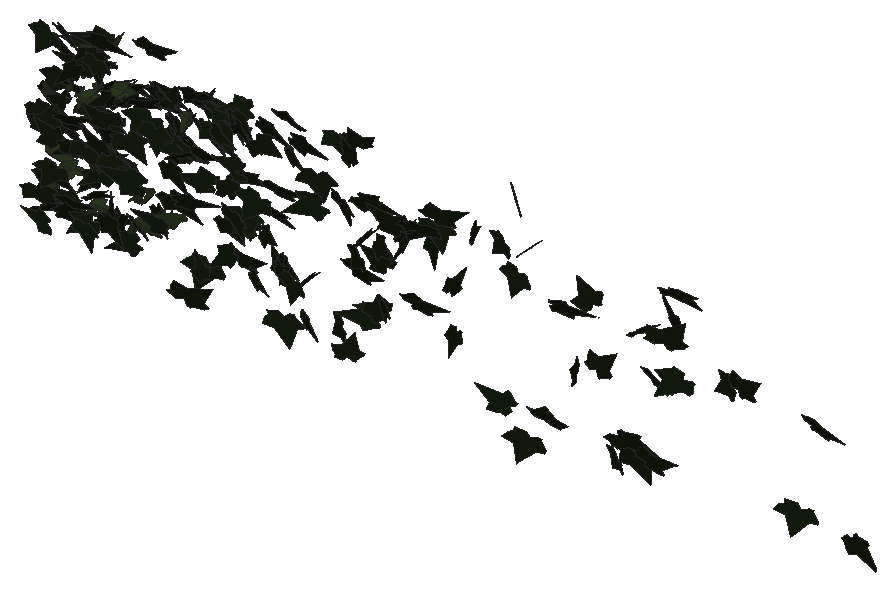
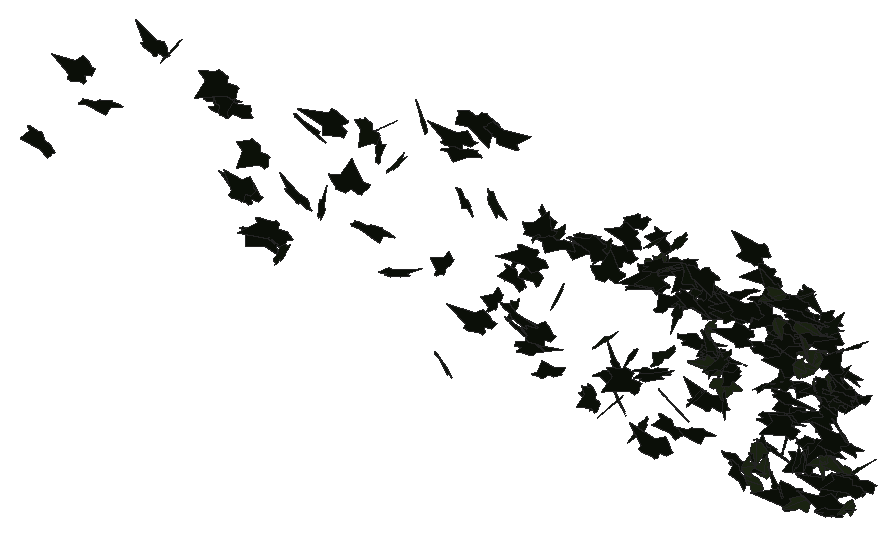
# SketchUp Ruby script. Lengths in millimetres.
U = 1.mm
M = Sketchup.active_model
def pt(a) = Geom::Point3d.new(a.map { |v| v * U })
def face(e, loops, mat)
  f = e.add_face(loops[0].map { |a| pt(a) })
  loops[1..].each { |l| e.add_face(l.map { |a| pt(a) }).erase! }
  f.material = f.back_material = mat if mat
  f
end
# faces: each face lists its corners as indices into pts; further lists are holes
def faces(e, pts, list, mat = nil) = list.each { |f| face(e, (f[0].is_a?(Array) ? f : [f]).map { |l| l.map { |i| pts[i] } }, mat) }
# xy, xz, yz: faces in a plane at the given z, y or x. An outline is a flat list of corners, or four numbers for a rectangle; further outlines are holes
def ring(l) = l.size == 4 ? [[l[0], l[1]], [l[2], l[1]], [l[2], l[3]], [l[0], l[3]]] : l.each_slice(2).to_a
def flat(e, list, mat, &to3) = list.each { |f| face(e, (f[0].is_a?(Array) ? f : [f]).map { |l| ring(l).map { |u, v| to3.(u, v) } }, mat) }
def xy(e, z, list, mat = nil) = flat(e, list, mat) { |x, y| [x, y, z] }
def xz(e, y, list, mat = nil) = flat(e, list, mat) { |x, z| [x, y, z] }
def yz(e, x, list, mat = nil) = flat(e, list, mat) { |y, z| [x, y, z] }
def lines(e, pts, list) = list.each { |a, b| e.add_line(pt(pts[a]), pt(pts[b])) }
# prism: a flat outline (further loops are holes) pulled along v
def prism(e, loops, v, mat = nil)
  f = face(e, loops, mat); d = Geom::Vector3d.new(v.map { |x| x * U })
  f.pushpull(f.normal.samedirection?(d) ? d.length : -d.length)
end
def box(e, o, s, mat = nil) = prism(e, [[o, [o[0] + s[0], o[1], o[2]], [o[0] + s[0], o[1] + s[1], o[2]], [o[0], o[1] + s[1], o[2]]]], [0, 0, s[2]], mat)
def at(x, y, z, deg = 0) = Geom::Transformation.translation(pt([x, y, z])) * Geom::Transformation.rotation(ORIGIN, Z_AXIS, deg.degrees)
def axes(o, x, y, z) = Geom::Transformation.new([*x, 0, *y, 0, *z, 0, *pt(o).to_a, 1])
def part(name) = M.definitions.add(name)
# library, detail: a bought-in or finely detailed component or shape, given as its bounding box
def library(name, o, s) = part(name).tap { |d| box(d.entities, o, s) }
def detail(e, o, s) = box(e.add_group.entities, o, s)
def put(e, d, t, mat = nil) = e.add_instance(d, t).tap { |i| i.material = mat if mat }
def group(e, t, mat = nil) = e.add_group.tap { |g| g.transformation = t; g.material = mat if mat }.entities
root = M.entities
M.materials.add("efeu1").color = [18, 25, 13]
M.materials.add("efeu2").color = [43, 57, 29]
c1 = part("ivyleaf_10")
p = [[0,12.8,-0.8],[-1.5,51.3,-10.9],[-4.9,51,-11.6],[-13.6,26.5,-7.3],[-13.2,15.9,-4.6],[-21.1,19.3,-7.2],
  [-29.5,16.3,-8.3],[-29.2,8.3,-6.2],[-19.7,-9.8,0.5],[-7.6,-13,4],[1,-12.2,5.8],[-0.4,51.1,-11.1],
  [-1.5,51.1,-10.9],[1,-12.4,5.9],[16.9,-12.4,3.5],[35.1,9.1,-5.1],[35,12.9,-6.1],[20.5,16.4,-4.9],
  [15.8,15,-3.8],[15.3,27.6,-7.1],[12.8,31.3,-7.8]]
faces(c1.entities,p,[[0,1,2,3,4,5,6,7,8,9,10],[11,12,0,13,14,15,16,17,18,19,20]],"efeu2")
c2 = part("ivyleaf_9")
p = [[39.1,54.8,31.7],[34.5,51.8,30.2],[-5.3,25.2,17.3],[-17.9,28.3,20.9],[-21.6,21.7,17],[-20.2,4.3,5.3],
  [-22.9,-0.3,2.5],[-17.1,-4,-0.6],[-2,-2.1,-1.2],[-0.7,-15.4,-10.1],[16.6,-22.3,-16.7],[21.1,-15.1,-12.5],
  [32.7,-10.7,-11],[46.1,-1.8,-6.6],[30.8,11.2,3.8]]
faces(c2.entities,p,[[0,1,2,3,4,5,6,7,8,9,10,11,12,13,14]],"efeu1")
put(root,c1,axes([6266.6,678.7,2682],[-0.03007,-0.47825,-1.14349],[0.82081,1.07001,-0.45348],[2.21157,-0.40363,0.15276]))
put(root,c2,axes([6279.4,678.7,3390.9],[-1.07005,-1.12342,0.65958],[-0.42506,-0.62463,-1.25427],[2.44266,-0.60083,0.07068]))
put(root,c2,axes([6295.3,729,3054],[-1.656,0.49645,-0.75374],[1.24652,-0.37303,-1.00177],[-1.18184,-1.08907,-0.00046]))
put(root,c2,axes([6319.9,714.5,3189.9],[-2.19819,-0.43278,-0.08904],[0.1664,0.02041,-1.23336],[0.82429,-1.15824,0.01153]))
put(root,c2,axes([6295.4,577.6,3112.4],[0.24045,-0.88792,-0.86385],[-0.29744,0.84997,-0.89651],[2.33887,0.19938,-0.0252]))
put(root,c2,axes([6275.2,666.3,2767.1],[-0.18875,-0.10741,-1.24219],[1.62396,0.90274,-0.14619],[1.73022,-0.85902,0.00169]))
put(root,c1,axes([6301.2,697.1,2840],[2.18033,0.00655,-0.47295],[0.89335,0.13694,1.13889],[0.1109,-1.23181,0.1241]))
put(root,c2,axes([6300.9,579.1,2737],[-0.72886,-0.55045,-1.10479],[1.2126,0.90257,-0.67055],[2.01201,-0.74336,0.00391]))
put(root,c2,axes([6364.8,718.6,2631.6],[-1.51195,-0.89067,-0.32702],[-0.41478,-0.24382,1.19349],[-1.75749,0.82378,-0.00034]))
put(root,c1,axes([6292.2,644.6,3145],[-0.32647,-0.02217,1.15106],[2.09254,-0.34829,0.15714],[0.64981,1.11043,0.07227]))
put(root,c2,axes([6346,717.7,3297.3],[1.4008,-0.87988,0.7248],[-0.72401,0.62372,1.14347],[-2.04522,-0.82344,0.09164]))
put(root,c2,axes([6297.5,715.3,2964.3],[2.07866,0.24286,-0.50673],[0.90485,0.19104,1.11629],[0.57008,-1.18877,0.07587]))
put(root,c2,axes([6308.1,647.3,3124.2],[-0.28171,-0.04101,1.39155],[1.28991,-1.22448,0.036],[2.31436,0.67748,0.14932]))
put(root,c1,axes([6387.1,673.7,3198.9],[0.05785,-0.09578,-1.24054],[-0.77272,1.17222,-0.10045],[2.23839,0.40714,-0.00262]))
put(root,c1,axes([6354.3,764.8,3350.5],[-0.66845,0.96883,-0.55194],[0.42948,-0.50494,-1.02992],[-2.07818,-0.41598,-0.03531]))
put(root,c2,axes([6356.7,534.3,2691.4],[1.49208,0.91629,0.52329],[0.5996,0.41892,-1.20553],[-1.91664,0.84438,0.03024]))
put(root,c2,axes([6350.2,644.9,3100.8],[-0.03128,-0.63876,0.97555],[0.48862,-0.95369,-0.62012],[2.1648,0.20603,0.15406]))
put(root,c1,axes([6378.4,715.9,2808.6],[-0.04611,-0.23692,-1.21513],[0.05876,-1.2151,0.2363],[-2.35544,-0.02568,0.02968]))
put(root,c2,axes([6394.5,660.2,3419.6],[0.93953,-1.17901,0.11255],[-0.0431,0.11251,1.27799],[-2.25369,-0.49367,0.02248]))
put(root,c2,axes([6403.1,569.7,2864.8],[-2.05259,-0.58279,-0.13758],[0.22938,0.06636,-1.22589],[1.11633,-1.08521,-0.00108]))
put(root,c2,axes([6420.2,703.2,2913.7],[-0.20926,0.13138,-1.23053],[-0.46783,-1.21308,-0.10755],[-2.30833,0.23395,0.13335]))
put(root,c2,axes([6354.4,692.6,3180.8],[2.05831,-0.25899,0.39907],[0.75322,-0.06023,-1.11163],[0.50248,1.1512,0.03162]))
put(root,c2,axes([6400,520,3067.7],[-2.29067,0.50467,0.62684],[1.1031,-0.23875,1.30511],[1.06252,1.33587,-0.00355]))
put(root,c2,axes([6355.1,690,2640.7],[0.70707,-0.36796,1.12674],[2.10631,-0.31509,-0.46782],[0.8077,1.1438,0.2336]))
put(root,c2,axes([6419.1,598.8,3154.3],[0.23842,0.1003,1.22912],[-1.70438,-0.84197,0.15998],[1.61359,-0.90416,-0.01263]))
put(root,c2,axes([6433.3,467.1,2672.7],[-0.08654,-1.34799,-0.04604],[0.00214,-0.0461,1.34876],[-2.56699,0.04541,0.00268]))
put(root,c1,axes([6386.6,657.2,2824.7],[0.39005,0.26603,1.22549],[1.30018,1.01763,-0.33515],[-2.00143,0.71292,0.02111]))
put(root,c2,axes([6431.5,700.9,2909.1],[2.01095,0.11688,-0.56713],[-1.07445,-0.05447,-1.06304],[-0.24507,1.19796,0.007]))
put(root,c1,axes([6422.2,704,3164.6],[1.17308,-0.80048,0.75418],[0.84602,-0.60946,-1.01016],[1.91454,0.75978,-0.01572]))
put(root,c1,axes([6452.1,746.8,3395.2],[1.1862,-0.92235,-0.47741],[-0.23757,0.48621,-1.10233],[1.96229,0.61642,0.15513]))
put(root,c2,axes([6481.9,722.5,3385.8],[-0.77989,-0.84585,-0.82752],[-0.61946,-0.76138,0.93943],[-2.16522,0.52249,0.0293]))
put(root,c2,axes([6436,754.9,3076.6],[-0.83453,-1.07187,-0.51547],[0.36246,0.47902,-1.15808],[2.23441,-0.47804,-0.00466]))
put(root,c1,axes([6442.5,684.8,3315],[1.72516,0.85466,0.04203],[0.04952,0.03367,-1.24582],[-1.62781,0.9068,0.00665]))
put(root,c2,axes([6464.9,710.4,2888.5],[0.75781,-0.24707,-1.11459],[-1.82015,0.57247,-0.46855],[1.18659,1.03592,-0.0069]))
put(root,c2,axes([6407,647.8,2993.7],[1.50874,-0.75455,0.87158],[1.22805,-0.58612,-1.09432],[1.81817,1.02203,0.01589]))
put(root,c2,axes([6411.6,587.8,2662.5],[0.80936,-0.05032,1.33235],[2.53752,0.01174,-0.42512],[0.00782,1.39852,0.0515]))
put(root,c2,axes([6510.3,428.8,3097.1],[-1.97137,0.20998,-0.75275],[-1.44439,0.02791,1.05209],[0.35485,1.28015,0.10053]))
put(root,c2,axes([6462.1,778.3,2838.9],[-0.05078,-0.40595,1.35296],[-0.3707,-1.33922,-0.40567],[2.66269,-0.19419,-0.03068]))
put(root,c2,axes([6447.7,543.2,2998.8],[-0.05441,0.04403,1.32423],[1.907,-0.86591,0.05042],[1.64989,1.0023,-0.01461]))
put(root,c1,axes([6468.6,734.1,2652.2],[-0.77778,-0.55874,-0.98942],[1.4926,0.62217,-0.67528],[1.5649,-0.87113,0.15232]))
put(root,c2,axes([6545.2,607,3347.3],[-0.41805,0.13574,1.32024],[-2.51658,0.09262,-0.22952],[-0.21707,-1.33518,0.1183]))
put(root,c1,axes([6526.1,661.9,3400.1],[-0.80222,-0.57488,0.96177],[-0.99064,-0.8095,-0.71199],[1.88844,-0.66886,0.03507]))
put(root,c2,axes([6517,545.2,3378],[-0.2312,0.01155,-1.42463],[1.01291,-1.32592,-0.05614],[-2.51515,-0.53504,0.10835]))
put(root,c2,axes([6564.4,683.5,3445.2],[-1.50148,0.19747,0.95868],[-1.81623,0.1186,-0.80975],[-0.41419,-1.23588,0.07547]))
put(root,c2,axes([6547.8,634.7,3410.6],[-0.05598,0.33739,-1.39931],[-0.27317,-1.39331,-0.33293],[-2.72583,0.1327,0.0621]))
put(root,c1,axes([6522.6,696.4,3225.9],[0.15412,-0.76268,1.01291],[0.45757,-0.98733,-0.76264],[2.36937,0.24028,0.08139]))
put(root,c2,axes([6547.2,636.9,2846.8],[-2.03528,0.35134,-0.41252],[0.73742,-0.14221,-1.12555],[-0.72092,-1.13735,0.01331]))
put(root,c2,axes([6565.5,585.4,2674.7],[-2.02022,-0.45335,0.24188],[-0.40697,-0.11504,-1.15405],[0.88923,-1.0826,0.02134]))
put(root,c1,axes([6510.7,632.9,3193.4],[0.3503,-0.05145,-1.16498],[1.94633,0.57386,0.13623],[1.06646,-1.03041,0.13404]))
put(root,c2,axes([6567.6,642.9,3375.6],[0.84076,0.97142,-0.69498],[-0.68628,-0.59796,-1.065],[-2.16717,0.56622,0.06763]))
put(root,c2,axes([6532.3,627.4,2761.6],[1.28845,0.66651,0.732],[0.97192,0.52458,-0.94994],[-1.61409,0.84791,0.01231]))
put(root,c2,axes([6609.1,702.3,3071.3],[-1.56562,0.22365,0.92477],[-1.67749,0.28117,-0.85205],[-0.6818,-1.20534,-0.02717]))
put(root,c1,axes([6573.3,761.8,3437.6],[0.06579,-1.20831,0.06088],[0.04827,-0.06017,-1.20858],[2.30208,0.0358,0.0236]))
put(root,c2,axes([6549.9,701.8,3231.7],[0.24967,0.98824,-0.75448],[0.06123,0.75571,0.99545],[2.36549,-0.12387,0.05387]))
put(root,c2,axes([6529.1,648.4,3468.7],[0.68088,0.26821,-1.29353],[2.09705,0.67868,0.44547],[1.38694,-1.15784,-0.03852]))
put(root,c2,axes([6532.1,701.5,2626.5],[1.59992,0.14641,1.21125],[2.24442,0.27959,-0.85226],[-0.59529,1.44763,0.0421]))
put(root,c2,axes([6555.4,426.8,3204.4],[1.94537,0.69503,-0.3976],[0.63124,0.21932,1.23606],[1.38705,-1.07461,-0.00488]))
put(root,c2,axes([6587.7,535.8,3047.2],[-0.83666,-0.94936,-0.81169],[0.61254,0.74534,-1.04607],[2.29692,-0.54457,-0.0167]))
put(root,c2,axes([6575.2,681.7,2934.6],[1.88559,0.49764,0.59362],[1.02041,0.25506,-1.10865],[-1.06405,1.12646,-0.01122]))
put(root,c2,axes([6591.3,515.6,2692.7],[0.0969,-1.32427,0.19587],[0.01365,-0.19574,-1.32525],[2.54773,0.05142,-0.00035]))
put(root,c2,axes([6643.4,585.4,2927],[-0.09201,-0.06097,-1.38196],[0.18702,-1.37946,0.05742],[-2.62605,-0.09611,0.05251]))
put(root,c2,axes([6609.5,708.1,2631.2],[-0.23895,0.49559,1.14591],[0.26713,-1.13879,0.50789],[2.36106,0.179,0.05851]))
put(root,c2,axes([6627.1,550,3437],[-0.32926,-1.2399,0.40661],[0.08316,-0.41544,-1.24824],[2.48203,-0.15056,0.09576]))
put(root,c2,axes([6669.9,604.3,3266.9],[-0.37121,-0.09302,-1.22697],[0.04772,-1.24233,0.0902],[-2.34139,-0.01057,0.19637]))
put(root,c2,axes([6714.3,656.3,2911.7],[-1.8155,-0.32988,1.04095],[-1.87957,-0.32911,-1.00931],[0.88671,-1.37303,-0.00816]))
put(root,c2,axes([6698.1,557.5,2743.6],[-0.25679,-0.5884,1.22047],[0.72283,1.16091,0.60167],[-2.47527,0.40005,0.04909]))
put(root,c2,axes([6709.6,560.3,3028.6],[-1.67467,-0.74934,0.47252],[-0.64155,-0.33269,-1.15531],[1.55919,-0.94173,0.03215]))
put(root,c2,axes([6682.7,553.6,3265.5],[0.47267,0.26229,1.23927],[1.261,1.04943,-0.35489],[-2.05473,0.70438,0.06728]))
put(root,c2,axes([6714.8,410.6,3374.2],[-1.13916,0.88865,-0.8294],[0.77499,-0.7245,-1.07012],[-2.1798,-0.72199,0.05298]))
put(root,c2,axes([6665.5,574.6,3065.7],[2.03694,-0.87994,-0.07632],[-0.10982,0.04999,-1.38556],[1.6774,1.07182,0.00197]))
put(root,c1,axes([6701.6,797.7,2752.2],[0.22388,-0.31093,1.16654],[0.54937,-1.13082,-0.33052],[2.23102,0.30966,-0.03567]))
put(root,c1,axes([6718.1,707.7,2800.5],[-0.45935,-1.16635,-0.4298],[0.1674,0.4207,-1.19106],[2.35979,-0.25688,0.00083]))
put(root,c2,axes([6745.9,421,3135.7],[0.40512,-0.39615,1.24207],[-1.29063,1.04122,0.44831],[-2.11915,-0.70987,-0.03558]))
put(root,c2,axes([6744.6,497.2,3185.7],[1.74975,0.46952,-1.02129],[-1.75093,-0.44374,-1.03219],[-1.22913,1.30052,0.01652]))
put(root,c1,axes([6732.2,650.2,2656.4],[-0.57653,-0.92854,-0.79827],[-0.22347,-0.79652,0.97106],[-2.31975,0.30751,0.10485]))
put(root,c1,axes([6706.9,729.7,2650.9],[-0.60067,0.08385,-1.18043],[2.0197,-0.52059,-0.32072],[-0.99671,-1.10544,0.0615]))
put(root,c2,axes([6708.2,768.5,3428],[0.03704,-0.26493,1.2844],[2.1284,-0.66759,-0.15465],[1.30368,1.09744,0.21599]))
put(root,c2,axes([6741.5,591.8,3347.2],[1.8339,0.79758,0.36569],[0.53628,0.23309,-1.25086],[-1.58145,1.00394,-0.00011]))
put(root,c2,axes([6804.1,401.3,3284.9],[0.64839,0.08173,1.27704],[-2.42801,0.12473,0.33236],[-0.18989,-1.3158,0.11083]))
put(root,c2,axes([6746.9,781.3,2703.9],[-0.58644,-0.04542,-1.39382],[2.6023,-0.29056,-0.29281],[-0.52196,-1.39759,0.10617]))
put(root,c2,axes([6764.5,629.9,2709.5],[1.54104,-0.82826,-0.57852],[0.85458,-0.36912,1.15692],[-1.72245,-0.92416,0.05641]))
put(root,c2,axes([6841.9,707.1,2693.4],[-0.93271,0.3241,1.15418],[-1.78096,0.67596,-0.58715],[-1.42613,-1.05611,-0.02161]))
put(root,c1,axes([6771.5,502.8,3384.9],[0.38468,0.50464,1.11578],[0.75701,1.0425,-0.54356],[-2.20427,0.44609,0.00805]))
put(root,c2,axes([6839.1,523.9,2695.7],[-2.21884,0.35783,0.27903],[-0.5125,0.07359,-1.21949],[-0.69508,-1.19651,0.00844]))
put(root,c2,axes([6770.5,515.4,3214.1],[0.52718,-0.84104,1.03036],[0.54819,-0.98956,-0.88517],[2.47125,0.39892,-0.02345]))
put(root,c2,axes([6791,550,2991.8],[0.00399,-1.203,-0.29037],[0.00829,0.29038,-1.20299],[2.35529,0.00102,0.00473]))
put(root,c2,axes([6791.3,495.9,3370.3],[0.74858,1.1447,0.66219],[-0.44457,-0.61986,1.21027],[2.47728,-0.45714,0.01709]))
put(root,c2,axes([6778.3,420.9,2830.9],[-0.51279,-0.07175,-1.46481],[2.79073,-0.03975,-0.26777],[-0.0498,-1.48886,0.07774]))
put(root,c2,axes([6835.2,720.2,3068.1],[-0.60733,-0.34503,1.1605],[1.43279,0.88335,0.46964],[-1.80457,0.81748,-0.01768]))
put(root,c2,axes([6790.8,687.6,3261.7],[1.65028,-0.31452,0.89042],[1.58751,-0.31165,-0.92237],[0.84261,1.20316,-0.00615]))
put(root,c2,axes([6848.4,745.5,3170],[1.7217,-1.06864,-0.39949],[-0.48324,0.30847,-1.40012],[2.11684,0.93958,0.0053]))
put(root,c2,axes([6937.9,421.2,3048],[-1.68127,-0.44861,-1.11531],[-1.85742,-0.54051,0.99041],[-1.3359,1.31611,0.02659]))
put(root,c2,axes([6898.6,543.9,3278.6],[-2.19944,-0.89341,0.10894],[-0.13315,-0.0876,-1.46049],[1.70775,-1.15747,0.02644]))
put(root,c2,axes([6845.7,651.2,3351.5],[0.29453,0.02861,-1.2753],[2.19728,0.54319,0.15228],[1.03247,-1.16417,0.03971]))
put(root,c2,axes([6870,423.5,3400.8],[0.12158,0.78312,-1.06902],[0.19885,1.06395,0.78566],[2.51422,-0.12202,-0.01044]))
put(root,c2,axes([6952.5,622.2,3334.8],[-0.53604,0.51474,1.17737],[-1.25313,0.97725,-0.58476],[-2.10012,-0.7145,0.04841]))
put(root,c2,axes([6873.4,665.3,3335.9],[1.47199,-0.98251,0.29118],[0.33531,-0.23187,-1.2504],[1.92126,0.79323,-0.00486]))
put(root,c2,axes([6909.2,698.6,3149.7],[-0.35525,0.93539,0.88445],[0.35091,-0.86506,0.95379],[2.42477,0.26223,-0.00846]))
put(root,c2,axes([6913.1,385.4,3265.6],[-0.4455,-0.97827,-1.00749],[0.50265,0.97249,-1.00565],[2.62495,-0.35225,0.02158]))
put(root,c2,axes([6963.4,703.4,3200.3],[-1.14986,0.68238,-1.01169],[-1.41902,0.68726,0.90882],[1.83859,0.95719,0.06871]))
put(root,c2,axes([6937.9,666.8,3116.8],[1.92428,-0.07908,-0.8091],[-1.44495,0.36981,-0.98489],[0.55318,1.24104,0.24192]))
put(root,c2,axes([6994,670.5,3105.4],[-1.764,-0.02912,0.90525],[-1.71011,-0.13313,-0.92428],[0.21651,-1.28873,0.07503]))
put(root,c2,axes([6955.2,622.3,2887.6],[-0.67434,0.30629,-1.39728],[2.11192,-0.84953,-0.46761],[-1.71798,-1.16456,-0.02638]))
put(root,c2,axes([6988.1,632.3,3104.6],[0.77425,1.19247,-0.27089],[-0.16795,-0.25611,-1.25996],[-2.32127,0.41628,0.00081]))
put(root,c1,axes([6975.3,688.4,3247.7],[-0.21939,-0.76405,1.00801],[0.69606,-0.98909,-0.70788],[2.30444,0.22601,0.30978]))
put(root,c1,axes([6947.2,692.6,3074.3],[0.28876,-0.20456,1.22546],[2.2054,0.46861,-0.06525],[-0.8529,1.14245,0.24618]))
put(root,c2,axes([6966.6,378.7,3438.9],[1.91667,0.87344,-0.11128],[0.14611,0.08132,1.33304],[1.66939,-1.00994,0.01109]))
put(root,c2,axes([6999.1,460.5,3297.4],[-0.75575,-1.2906,-0.0785],[0.0477,0.07442,-1.35031],[2.46035,-0.39788,0.00207]))
put(root,c1,axes([7039.9,516.9,2893.9],[-1.89203,-0.79052,-0.06912],[0.10364,0.04258,-1.27013],[1.50671,-0.99562,0.00056]))
put(root,c2,axes([7107.3,688.8,3346.7],[-0.45534,-0.04646,-1.29065],[-2.4303,-0.18787,0.24347],[-0.36774,1.29913,-0.01094]))
put(root,c2,axes([7081.7,611.2,3429.5],[1.19843,0.60238,-0.88819],[-1.33218,-0.55008,-0.86932],[-1.54826,0.93958,0.06049]))
put(root,c2,axes([7044,502.8,2991],[-0.25942,-0.21723,-1.44326],[2.44179,0.6732,-0.2225],[1.32423,-1.28389,0.12753]))
put(root,c2,axes([7120.2,616.3,3398.5],[0.51569,0.53541,1.09573],[0.54391,1.06331,-0.59025],[-2.2564,0.37868,0.10814]))
put(root,c2,axes([7178,574.4,3064.2],[-1.16004,-0.00036,1.19221],[-2.26471,-0.08215,-0.60839],[0.13952,-1.33646,0.03708]))
put(root,c2,axes([7120,615.2,3393.7],[2.23292,0.42953,-0.0039],[-0.01872,0.01552,-1.24927],[-0.8173,1.17315,0.01795]))
put(root,c2,axes([7104.4,764.3,2788],[-0.35243,-0.11555,-1.22632],[2.30548,0.20757,-0.20248],[0.42468,-1.22273,0.08152]))
put(root,c2,axes([7149.8,599.6,2677.4],[-2.00538,-1.03255,-0.1616],[0.21176,0.11735,-1.47526],[1.97777,-1.05953,-0.0059]))
put(root,c2,axes([7114.8,608.8,3296.2],[1.52852,-1.25451,-0.12099],[-0.11823,0.10389,-1.48957],[2.39576,0.80552,0.00369]))
put(root,c2,axes([7112.4,399.5,3197.3],[-0.48874,-0.10479,-1.39468],[2.65819,0.05486,-0.26129],[0.13905,-1.41706,0.09302]))
put(root,c2,axes([7171.1,637.4,3234.8],[1.29751,-0.29692,-1.08173],[-1.75424,0.57315,-0.73824],[1.21672,1.14299,0.08918]))
put(root,c2,axes([7156.3,488.3,3257],[0.4193,-0.5165,1.38292],[1.59856,-1.10599,-0.54688],[2.31045,0.85895,0.12741]))
put(root,c2,axes([7217,629.4,3390.9],[-1.25519,-1.09232,0.3337],[-0.33998,-0.28195,-1.27596],[2.14701,-0.68324,-0.00696]))
put(root,c2,axes([7238.7,461.8,2718],[-0.85068,-0.88498,0.81564],[0.68442,0.73212,0.99142],[-2.1859,0.57363,-0.007]))
put(root,c2,axes([7181.3,758.1,2640.5],[-0.12809,-0.27756,1.4356],[2.02171,-0.99684,-0.14293],[1.9123,1.03528,0.24727]))
put(root,c2,axes([7281.9,584.2,2778.1],[-2.32726,0.66405,-0.36378],[0.58704,-0.19418,-1.3913],[-1.31604,-1.26091,0.02268]))
put(root,c2,axes([7211,352.9,3091.9],[1.13476,-0.00277,1.21045],[2.29706,0.10396,-0.59428],[-0.17516,1.34531,0.04842]))
put(root,c2,axes([7294.6,667.1,3401.9],[-1.04582,-0.37194,1.16968],[-1.81109,-0.68032,-0.66338],[1.47539,-1.09876,0.0148]))
put(root,c2,axes([7230.3,359,2655.9],[-0.93498,0.04059,1.4223],[2.34728,-0.7382,0.44707],[1.35043,1.31123,0.20766]))
put(root,c2,axes([7256.3,521.7,3375.1],[-0.43572,-1.17344,-0.9063],[0.26966,0.89553,-1.19529],[2.80893,-0.268,-0.02584]))
put(root,c2,axes([7331.4,658.7,2878.7],[-1.51868,-1.07819,-0.15225],[-0.10437,-0.14873,1.34063],[-2.06974,0.79862,0.04412]))
put(root,c2,axes([7288.5,661.6,2931.1],[-0.94399,-1.10169,-0.50895],[0.49363,0.44088,-1.20712],[2.2563,-0.55738,0.05116]))
put(root,c1,axes([7315.9,587.8,3349.8],[-1.83022,-0.72892,-0.38434],[-0.5638,-0.24538,1.20658],[-1.46346,1.00612,0.01582]))
put(root,c2,axes([7273.6,621.7,3327.7],[1.93084,-0.84116,0.1064],[0.17266,-0.05727,-1.31781],[1.60438,1.01848,0.01377]))
put(root,c2,axes([7281.3,593.8,2955.1],[0.38998,-1.34864,0.64485],[0.26488,-0.63084,-1.36357],[2.8327,0.24466,0.03873]))
put(root,c2,axes([7294.8,591.4,3356.4],[0.32503,-0.82121,0.94718],[0.27992,-0.9362,-0.83821],[2.36939,0.22326,-0.03091]))
put(root,c2,axes([7310.8,439.2,3416.1],[1.69245,-0.64732,-0.83166],[-0.92341,0.71453,-1.07495],[1.78056,0.98585,0.23303]))
put(root,c2,axes([7327.4,661,2665.2],[1.51487,-0.77627,-0.72363],[-1.00681,0.49392,-1.11174],[1.75093,0.95563,-0.0132]))
put(root,c2,axes([7346.2,484,3125.1],[-1.00222,-0.48738,1.32358],[1.80762,0.92196,0.71737],[-1.98457,1.08589,-0.01501]))
put(root,c2,axes([7321.6,759.6,2920.5],[2.66001,0.03322,0.01958],[0.03654,0.01629,-1.39796],[-0.06365,1.39769,0.01583]))
put(root,c2,axes([7339.9,540,3455.9],[0.8936,-1.24017,-0.27419],[-0.18871,0.25564,-1.32607],[2.40991,0.47988,-0.00217]))
put(root,c2,axes([7406.7,486.5,3251.1],[-0.07648,-1.39427,-0.33401],[0.03223,-0.33458,1.39461],[-2.72846,0.03513,0.02584]))
put(root,c2,axes([7348.2,511.8,3435.8],[0.00662,0.00623,-1.3074],[2.48559,-0.06071,0.00318],[-0.11551,-1.306,-0.00639]))
put(root,c2,axes([7447.8,674.1,2740],[-0.15308,0.44334,1.26449],[-0.24225,1.25851,-0.44934],[-2.53868,-0.14683,-0.03337]))
put(root,c2,axes([7421.3,766.4,3353.7],[2.24101,-0.62437,0.12941],[-0.20927,0.06886,1.33276],[-1.19538,-1.18258,0.00928]))
put(root,c2,axes([7435.4,596,2926],[0.82153,-0.46621,-1.10809],[-1.28036,0.88207,-0.63318],[1.89617,0.79759,0.05255]))
put(root,c2,axes([7399.4,476.9,3220.8],[2.23649,0.32103,0.82368],[1.52436,0.19327,-1.21801],[-0.71211,1.42197,-0.02041]))
put(root,c2,axes([7439.2,691.3,2750.5],[1.15747,-0.66893,-0.96136],[-0.86999,0.86175,-0.88881],[2.05222,0.74261,0.16543]))
put(root,c2,axes([7509.7,472.7,3154.6],[-1.51415,-1.14656,0.49012],[-0.43445,-0.43763,-1.39432],[2.33303,-0.82562,0.05844]))
put(root,c2,axes([7456.9,568.9,3436.8],[0.55535,0.06799,-1.39788],[2.65222,0.11773,0.29662],[0.24593,-1.42315,-0.04225]))
put(root,c2,axes([7526.7,444.6,3438.7],[0.34739,-0.45456,-1.30556],[-0.35981,1.29631,-0.47778],[2.60633,0.23955,0.10806]))
put(root,c2,axes([7555.4,548.4,2789.9],[-0.3404,0.60802,1.17923],[0.17864,-1.18111,0.62323],[2.51874,0.16594,0.11517]))
put(root,c2,axes([7572.1,675.6,2705.9],[0.58548,0.62151,1.16267],[0.99927,1.03738,-0.69346],[-2.30154,0.60851,-0.00531]))
put(root,c2,axes([7575.1,581,3353.3],[1.57919,-0.82381,-0.73705],[-1.05243,0.48863,-1.16869],[1.82163,0.99648,-0.03625]))
put(root,c2,axes([7564.9,639.8,3371.3],[1.02379,-0.026,-1.2387],[2.29194,0.32843,0.51608],[0.55432,-1.30992,0.15398]))
put(root,c2,axes([7602.5,461.3,3233.8],[0.17772,-0.55313,1.27344],[2.26452,-0.62581,-0.35908],[1.36162,1.11298,0.43097]))
put(root,c2,axes([7668,434.9,2688.3],[-0.80698,-1.40267,-0.37145],[0.28719,0.34226,-1.4647],[2.74661,-0.4479,0.04401]))
put(root,c2,axes([7682,477.7,2837.6],[-0.33278,-1.21944,0.77996],[-0.20247,-0.77268,-1.2319],[2.7475,-0.20464,0.00369]))
put(root,c2,axes([7663.1,568.7,2636.2],[0.10214,-0.00351,-1.34428],[2.46826,-0.3539,0.0527],[-0.67327,-1.29797,-0.01074]))
put(root,c2,axes([7714.4,731,3397.9],[-1.12271,-0.77371,-0.86052],[0.98585,0.68716,-0.97294],[1.96944,-0.78504,-0.00353]))
put(root,c2,axes([7728.4,570.8,3297.4],[-1.37445,-0.88228,-0.72869],[0.8655,0.56942,-1.14013],[1.99845,-0.8534,-0.00738]))
put(root,c2,axes([7828.8,451.3,3250.1],[-2.14018,-0.46434,0.75827],[-1.33543,-0.28743,-1.21661],[1.03934,-1.32548,-0.00181]))
put(root,c2,axes([7810.8,724.6,3397],[1.36346,0.40979,1.01249],[-1.85375,-0.3083,0.81397],[0.94079,-1.20138,0.13648]))
put(root,c2,axes([7857.4,620.8,3389.3],[0.15751,-0.05246,1.38006],[-0.50133,1.35655,0.06737],[-2.58016,-0.26678,0.07116]))
put(root,c2,axes([7850.9,653.2,2873.1],[0.42018,-0.35198,1.40349],[1.81317,-1.03321,-0.40898],[2.07269,0.9752,0.07326]))
put(root,c2,axes([7885.4,527.9,3256.7],[0.36713,-1.20407,0.89151],[0.26132,-0.88088,-1.21942],[2.83936,0.23676,-0.00304]))
put(root,c2,axes([7898.3,642.4,3220.7],[0.37276,0.22557,-1.35132],[1.63138,1.04469,0.29862],[2.03401,-0.87923,0.00813]))
put(root,c2,axes([7995.9,666,2939.2],[-0.5665,0.50802,1.2762],[-1.46667,1.01919,-0.58545],[-2.16404,-0.82374,0.06271]))
put(root,c2,axes([7955.6,483.8,2597.6],[-1.4628,-0.37262,0.95698],[1.61464,0.44319,0.85395],[-1.10139,1.14461,-0.01911]))
put(root,c2,axes([8009,576.9,2740.6],[-1.23641,-0.15523,1.24591],[-2.25016,-0.39649,-0.66588],[0.80421,-1.34801,0.05238]))
put(root,c2,axes([7931.7,715.6,3153.6],[-0.3687,-0.06228,-1.29895],[2.47143,0.06138,-0.19661],[0.13315,-1.31189,0.05247]))
put(root,c2,axes([7963.2,546.7,3092],[0.63919,0.5858,1.30395],[1.15803,1.15347,-0.67492],[-2.46185,0.69468,0.02108]))
put(root,c2,axes([8007,751.3,3026.1],[-0.21802,-0.06879,1.32131],[1.5497,1.04169,0.12482],[-1.98478,0.8209,-0.04768]))
put(root,c2,axes([8078.7,551.7,2809],[-1.65886,0.87263,0.69734],[-0.94861,0.48775,-1.23335],[-1.90257,-1.00404,0.00693]))
put(root,c2,axes([8044.4,331,2823.7],[-0.28538,-0.40476,1.41284],[-0.70817,-1.36345,-0.4301],[2.70596,-0.39951,0.03644]))
put(root,c2,axes([8060.2,540.5,3121.3],[1.00127,-0.7021,-1.18884],[-1.43819,0.91834,-0.87675],[2.19921,0.92021,-0.03209]))
put(root,c2,axes([8088.3,383.5,3136.2],[-0.36742,-0.65064,1.1755],[-0.36943,-1.16161,-0.67482],[2.53022,-0.26408,0.07217]))
put(root,c2,axes([8090,532.6,2863.2],[0.7391,-0.25591,-1.24287],[1.88356,-0.75241,0.46416],[-1.51153,-1.06274,-0.02933]))
put(root,c2,axes([8152.4,657.4,2825.8],[0.568,-0.35075,1.32122],[2.22402,-0.63624,-0.43286],[1.34993,1.19579,0.15723]))
put(root,c2,axes([8269.7,774,2681],[-1.69806,0.31655,-0.96952],[1.73487,-0.33024,-0.94669],[-0.87058,-1.27552,0.00449]))
put(root,c2,axes([8291.9,428.8,3255.6],[-1.5848,0.72894,-1.02479],[1.40718,-0.71045,-1.10613],[-1.9361,-1.11303,0.0349]))
put(root,c2,axes([8391.1,256.6,3423.1],[0.18497,-0.04628,1.45505],[-2.34527,0.77382,0.10692],[-1.47518,-1.23604,0.01246]))
put(root,c2,axes([8381.4,606.4,2992.1],[-0.33562,-0.26448,1.37965],[1.67637,1.06237,0.31624],[-2.08272,0.89772,0.03222]))
put(root,c2,axes([8373.6,496.5,3258.6],[-1.23922,0.17954,-1.23752],[2.27808,-0.31427,-0.67539],[-0.68871,-1.36259,-0.00729]))
put(root,c2,axes([8463.6,403.6,3403.8],[-1.1724,-1.03523,-0.66624],[0.71053,0.55282,-1.20419],[2.23268,-0.71954,0.03337]))
put(root,c2,axes([8501.9,255.6,3474.7],[1.38552,0.85294,-0.96205],[-1.19609,-0.72842,-1.12137],[-2.13471,0.96173,0.0039]))
put(root,c2,axes([8463.4,403.5,3436.5],[-0.35137,0.07935,1.36237],[2.5255,-0.3105,0.19791],[0.60632,1.33931,-0.03484]))
put(root,c2,axes([8676.9,667.6,3428.1],[-0.03443,-0.69878,1.18156],[0.17538,1.17838,0.69831],[-2.60668,0.08851,0.03138]))
put(root,c2,axes([8658.8,388.7,3431.2],[0.21395,0.72856,1.12827],[-0.25469,-1.12051,0.73688],[2.54338,-0.17349,-0.02112]))
put(root,c2,axes([8674.1,567.9,3323.2],[-0.63917,-0.6519,1.17848],[-0.47349,-1.16363,-0.71459],[2.51906,-0.38413,0.1647]))
put(root,c2,axes([8829.5,399.7,2716.3],[-1.62744,-0.99666,-0.29529],[-0.36669,-0.22378,1.31322],[-1.94408,0.87655,-0.0005]))
put(root,c2,axes([8856.4,479.4,3388.3],[0.74353,0.99458,1.02562],[0.5758,0.98157,-1.0671],[-2.65738,0.49097,0.05575]))
put(root,c2,axes([8895,385,3340.1],[-0.66403,-1.28927,0.65454],[-0.2358,-0.64419,-1.33493],[2.74173,-0.36766,0.04372]))
put(root,c2,axes([9099.1,200.3,2744.9],[-2.37959,-0.62231,-0.41862],[0.71368,0.18608,-1.39662],[1.2362,-1.30533,0.00048]))
put(root,c2,axes([9115.7,477.4,2923.1],[0.17077,0.22298,1.4847],[-0.97296,-1.39393,0.24025],[2.68661,-0.51898,-0.00737]))
put(root,c2,axes([9207.3,463.1,3284.6],[-2.39329,0.45835,-0.70147],[-1.27792,0.2056,1.33804],[0.95406,1.42518,0.03257]))
put(root,c2,axes([9110.4,367.9,3277.3],[1.49496,0.53092,-1.0637],[1.68813,0.58715,0.94807],[1.5065,-1.18479,-0.00682]))
put(root,c2,axes([9198.6,180.4,2878.4],[2.56373,-0.46156,0.34499],[-0.572,0.18566,1.42191],[-0.93573,-1.37809,0.07601]))
put(root,c2,axes([9198.3,509.2,2961.8],[-0.99971,0.8642,1.07558],[1.03218,-0.92893,1.01123],[2.41458,0.7549,0.01305]))
put(root,c2,axes([9343,453.4,2628.2],[-0.29835,-0.55458,1.34874],[-0.28455,-1.34325,-0.5697],[2.76082,-0.19838,0.08703]))
put(root,c2,axes([9352.4,577,3158.2],[1.40139,1.00964,0.83519],[0.86482,0.70182,-1.24903],[-2.33903,0.86439,0.03858]))
put(root,c2,axes([9369.4,443.5,2743.7],[-0.01746,0.07122,-1.46837],[1.71846,1.15906,0.05058],[2.20795,-0.90154,-0.05098]))
put(root,c2,axes([9417.5,588.7,2955.7],[0.35223,-0.69155,1.3362],[1.16268,-1.19576,-0.70348],[2.61679,0.62438,0.1327]))
put(root,c2,axes([9443.9,448.5,2687.8],[-1.3875,-0.404,-1.21646],[2.13778,0.47281,-0.8302],[1.1752,-1.33706,0.07399]))
put(root,c2,axes([9577.6,540.1,3276.7],[0.16609,-0.54139,1.41505],[-0.46942,1.39341,0.54832],[-2.84504,-0.26151,-0.00786]))
put(root,c2,axes([9529.4,564.4,3406],[2.78417,0.34522,0.16055],[0.29688,0.03799,-1.50307],[-0.66099,1.47118,0.00114]))
put(root,c2,axes([9560,481.6,3222.7],[-1.54739,-0.08015,1.26785],[2.4056,-0.20199,0.79779],[0.24246,1.49254,0.17605]))
put(root,c2,axes([9595,329.6,2760.1],[0.14596,-0.0126,1.4292],[1.95115,-0.99677,-0.0638],[1.89533,1.0271,-0.04438]))
put(root,c2,axes([9750.3,356.5,3172],[-2.44674,-0.62066,0.25406],[-0.40361,-0.14489,-1.42708],[1.21089,-1.30242,0.03768]))
put(root,c2,axes([10018.8,329,3250.1],[-0.6848,-0.41985,1.36113],[-0.8604,-1.29764,-0.51977],[2.57078,-0.54614,0.18862]))
put(root,c2,axes([10071.1,323.3,3257.3],[-0.59834,0.32855,1.40055],[1.38861,-1.19911,0.44508],[2.35961,0.78898,0.09322]))
put(root,c2,axes([10334.5,463.6,3119.8],[0.96918,-0.68949,1.23167],[1.58724,-0.90943,-0.85391],[2.16739,0.97431,0.07458]))
put(root,c2,axes([10435.3,252.5,2865.6],[-1.88218,-1.09487,-0.20165],[0.26465,0.14613,-1.47538],[2.10221,-0.99867,0.00519]))
put(root,c2,axes([10581.3,411,2709.2],[-0.42755,-0.18231,-1.48321],[2.82074,0.16459,-0.24471],[0.36365,-1.49107,0.15434]))
